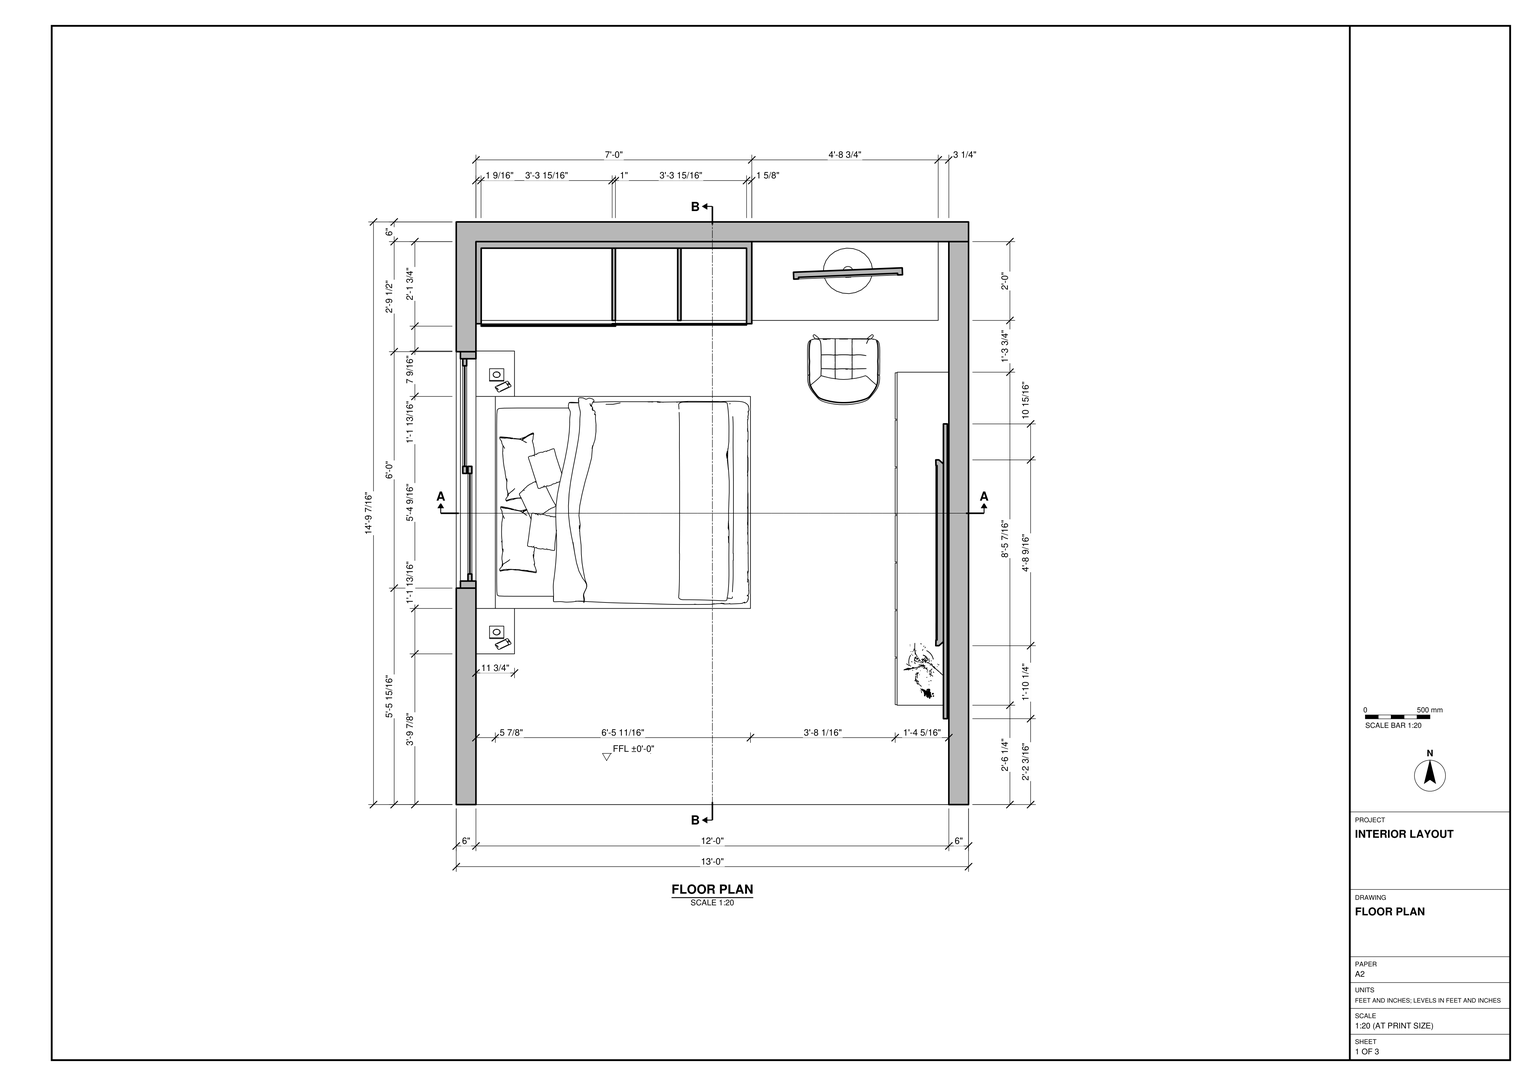
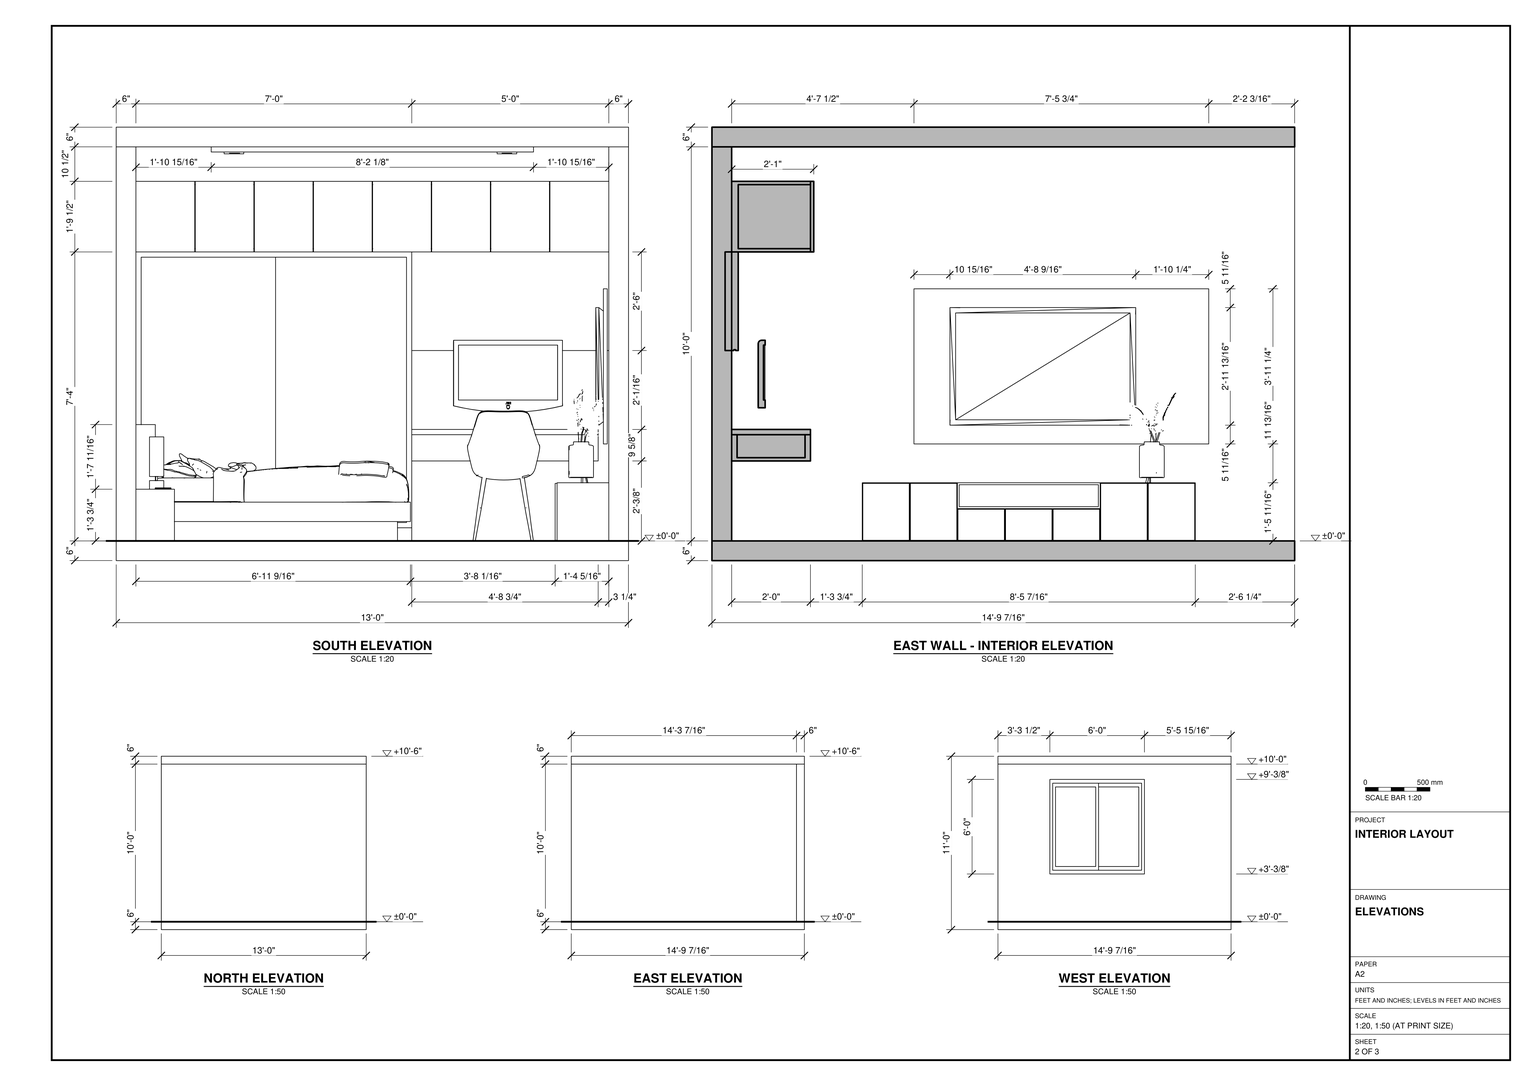
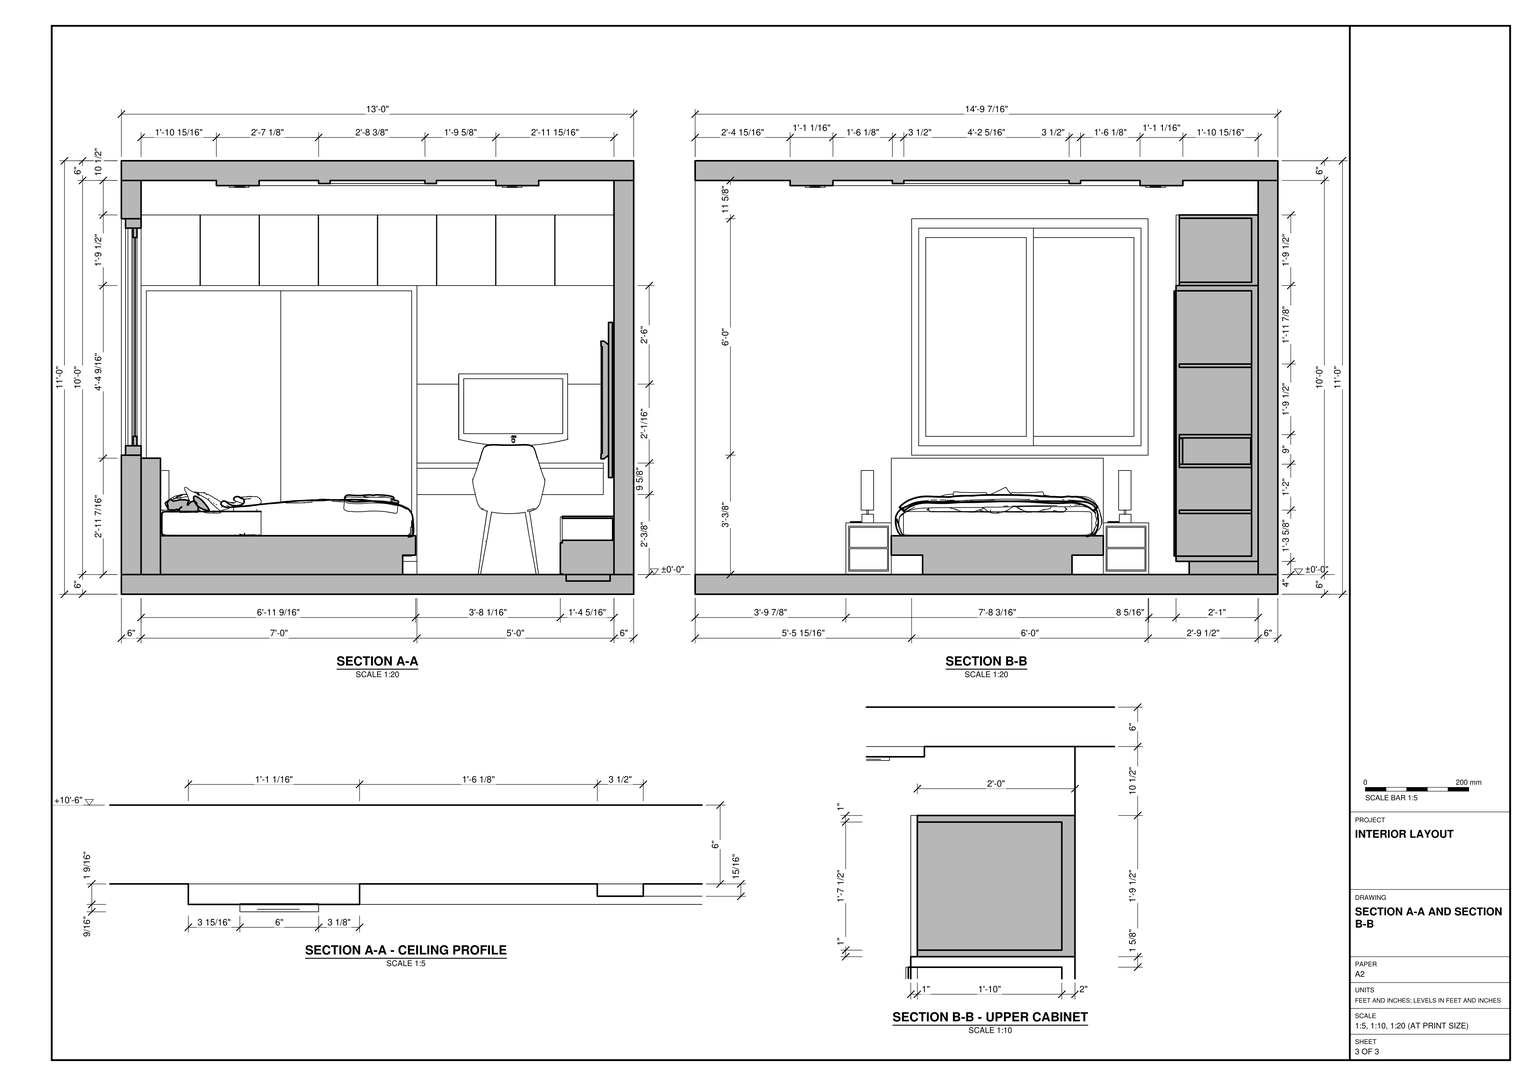
Build the bedroom interior in SketchUp from task_files/diagram_01.pdf. Work in feet and inches. Use the floor plan to set out the room and the elevations and sections to establish heights. The overall dimensions are 13'-0" east to west, 14'-9 7/16" north to south and 11'-0" high. Set the finished floor at ±0'-0". Model the floor slab, the north, east and west walls, and the flat roof slab, leaving the south side open as drawn. Follow the enlarged section for the stepped ceiling profile.

Place the head of the platform bed beneath the framed west window, with a bedside table on either side. Along the north wall, fit the tall wardrobe beside the desk and continue the upper cabinets across both. Include the desk screen and chair. Across the aisle from the foot of the bed, model the east-wall television, its backing panel and the low divided cabinet beneath it. Use the plan for the furniture footprints and the interior elevations for the cabinet divisions. Decor and loose items, including bedside lamps, cushions and the arrangement on the low cabinet, may be any suitable library components.

Keep shell elements and individual furniture and joinery pieces in separate groups or components, and use components for repeated parts. Save one SketchUp model as output_files/bedroom_with_fitted_storage_desk_and_television_wall.skp.

# SketchUp Ruby script. Lengths in inches.
U = 1.inch
M = Sketchup.active_model
def pt(a) = Geom::Point3d.new(a.map { |v| v * U })
def face(e, loops, mat)
  f = e.add_face(loops[0].map { |a| pt(a) })
  loops[1..].each { |l| e.add_face(l.map { |a| pt(a) }).erase! }
  f.material = f.back_material = mat if mat
  f
end
# faces: each face lists its corners as indices into pts; further lists are holes
def faces(e, pts, list, mat = nil) = list.each { |f| face(e, (f[0].is_a?(Array) ? f : [f]).map { |l| l.map { |i| pts[i] } }, mat) }
# xy, xz, yz: faces in a plane at the given z, y or x. An outline is a flat list of corners, or four numbers for a rectangle; further outlines are holes
def ring(l) = l.size == 4 ? [[l[0], l[1]], [l[2], l[1]], [l[2], l[3]], [l[0], l[3]]] : l.each_slice(2).to_a
def flat(e, list, mat, &to3) = list.each { |f| face(e, (f[0].is_a?(Array) ? f : [f]).map { |l| ring(l).map { |u, v| to3.(u, v) } }, mat) }
def xy(e, z, list, mat = nil) = flat(e, list, mat) { |x, y| [x, y, z] }
def xz(e, y, list, mat = nil) = flat(e, list, mat) { |x, z| [x, y, z] }
def yz(e, x, list, mat = nil) = flat(e, list, mat) { |y, z| [x, y, z] }
def lines(e, pts, list) = list.each { |a, b| e.add_line(pt(pts[a]), pt(pts[b])) }
# prism: a flat outline (further loops are holes) pulled along v
def prism(e, loops, v, mat = nil)
  f = face(e, loops, mat); d = Geom::Vector3d.new(v.map { |x| x * U })
  f.pushpull(f.normal.samedirection?(d) ? d.length : -d.length)
end
def box(e, o, s, mat = nil) = prism(e, [[o, [o[0] + s[0], o[1], o[2]], [o[0] + s[0], o[1] + s[1], o[2]], [o[0], o[1] + s[1], o[2]]]], [0, 0, s[2]], mat)
def at(x, y, z, deg = 0) = Geom::Transformation.translation(pt([x, y, z])) * Geom::Transformation.rotation(ORIGIN, Z_AXIS, deg.degrees)
def axes(o, x, y, z) = Geom::Transformation.new([*x, 0, *y, 0, *z, 0, *pt(o).to_a, 1])
def part(name) = M.definitions.add(name)
# library, detail: a bought-in or finely detailed component or shape, given as its bounding box
def library(name, o, s) = part(name).tap { |d| box(d.entities, o, s) }
def detail(e, o, s) = box(e.add_group.entities, o, s)
def put(e, d, t, mat = nil) = e.add_instance(d, t).tap { |i| i.material = mat if mat }
def group(e, t, mat = nil) = e.add_group.tap { |g| g.transformation = t; g.material = mat if mat }.entities
root = M.entities
M.materials.add("[0005_LightPink]").color = [189, 180, 163]
M.materials.add("[0057_DarkKhaki]").color = [189, 183, 107]
M.materials.add("[0092_Azure]").color = [90, 107, 113]
M.materials.add("[Color A01]").color = [96, 100, 74]
M.materials.add("[Color A03]").color = [146, 98, 60]
M.materials.add("[Color A03]1").color = [255, 101, 101]
M.materials.add("[Color H07]").color = [0, 153, 153]
M.materials.add("[Color H08]").color = [0, 102, 102]
M.materials.add("[Color M00]").color = [255, 255, 255]
M.materials.add("[CoolGray4]").color = [225, 226, 230]
M.materials["[CoolGray4]"].alpha = 0.26
M.materials.add("[Field Square Tile]").color = [217, 201, 169]
M.materials.add("[Mirror 02]").color = [229, 229, 229]
M.materials.add("[Roofing Slate Tan]").color = [200, 175, 128]
M.materials.add("[Translucent Glass Blue]").color = [100, 149, 237]
M.materials["[Translucent Glass Blue]"].alpha = 0.5
M.materials.add("[Wood Bamboo]").color = [177, 105, 43]
M.materials.add("[Wood Cherry Original]1").color = [152, 86, 42]
M.materials.add("[Wood Veneer 02]").color = [190, 128, 91]
c1 = part("Cabinet shelf")
box(c1.entities,[0,0,0],[39.93,22,1])
c2 = part("Drawer box")
g1 = group(c2.entities,at(0,1.6875,0))
xy(g1,0,[[0,0,0,22,1,22,1,1,18.96,1,18.96,22,19.96,22,19.96,0],[1,21.75,18.96,22]],"[Wood Veneer 02]")
xy(g1,7.625,[[1,21.75,18.96,22]],"[Wood Veneer 02]")
xy(g1,7.8125,[[0,0,19.96,0,19.96,22,18.96,22,18.96,1,1,1,1,22,0,22]],"[Wood Veneer 02]")
xz(g1,0,[[0,0,19.96,7.8125]],"[Wood Veneer 02]")
xz(g1,1,[[1,0,18.96,7.8125]],"[Wood Veneer 02]")
xz(g1,21.75,[[1,0,18.96,7.625]],"[Wood Veneer 02]")
xz(g1,22,[[0,0,1,7.8125],[1,0,18.96,7.625],[18.96,0,19.96,7.8125]],"[Wood Veneer 02]")
yz(g1,0,[[0,0,22,7.8125]],"[Wood Veneer 02]")
yz(g1,1,[[1,0,21.75,7.8125],[21.75,0,22,7.625],[21.75,7.625,22,7.8125]],"[Wood Veneer 02]")
yz(g1,18.96,[[1,0,21.75,7.8125],[21.75,0,22,7.625],[21.75,7.625,22,7.8125]],"[Wood Veneer 02]")
yz(g1,19.96,[[0,0,22,7.8125]],"[Wood Veneer 02]")
c3 = library("pc",[0,0,0],[196.92,471.66,385.83])
c4 = part("Component")
put(c4.entities,c3,at(-98.46,-353.84,0))
c5 = library("1",[-11,-10.66,0],[22,21.32,33.52])
c6 = library("1.1 TV UNIT",[4.49,5.68,0],[124.23,70.56,78.75])
c7 = library("Double bed",[0,0,0],[83.59,112.46,35.43])
c8 = library("Component\#7",[0,0,0],[6,6,0.625])
c9 = part("Window sash")
g2 = group(c9.entities,at(0.98,0,0))
prism(g2,[[[-0.98,0,0],[30.98,0,0],[30.98,0,45.6],[-0.98,0,45.6]],[[29.01,0,43.625],[29.01,0,1.97],[0.98,0,1.97],[0.98,0,43.625]]],[0,1.18,0])
g3 = group(c9.entities,at(1.97,0.59,1.97),"[Translucent Glass Blue]")
xz(g3,0,[[0,0,28.03,41.66]],"[CoolGray4]")
c10 = part("Two-panel window")
put(c10.entities,c9,at(31.97,2.82,1.97),"[Wood Bamboo]")
put(c10.entities,c9,at(1.97,1.25,1.97),"[Wood Bamboo]")
g4 = group(c10.entities,at(0,0,0),"[Wood Bamboo]")
prism(g4,[[[65.9,4.72,0],[0,4.72,0],[0,4.72,49.53],[65.9,4.72,49.53]],[[1.97,4.72,47.5625],[1.97,4.72,1.97],[63.93,4.72,1.97],[63.93,4.72,47.5625]]],[0,-4.72,0])
c11 = part("Union")
prism(c11.entities,[[[39.93,0,21.5],[19.96,0,21.5],[19.96,0,43.8],[18.96,0,43.8],[18.96,0,21.5],[0,0,21.5],[0,0,20.5],[18.96,0,20.5],[18.96,0,0],[19.96,0,0],[19.96,0,20.5],[39.93,0,20.5]]],[0,22,0])
c12 = part("Group\#17")
box(c12.entities,[-1,0,0],[1,22,19.5])
c13 = part("Drawer box \#1")
xy(c13.entities,0,[[0,0,29.3125,14.5]])
xy(c13.entities,1,[[1,1,28.125,13.5]])
xy(c13.entities,8,[[[0,0,29.3125,14.5],[1,1,28.125,13.5]]])
xz(c13.entities,0,[[0,0,29.3125,8]])
xz(c13.entities,1,[[1,1,28.125,8]])
xz(c13.entities,13.5,[[1,1,28.125,8]])
xz(c13.entities,14.5,[[0,0,29.3125,8]])
yz(c13.entities,0,[[0,0,14.5,8]])
yz(c13.entities,1,[[1,1,13.5,8]])
yz(c13.entities,28.125,[[1,1,13.5,8]])
yz(c13.entities,29.3125,[[0,0,14.5,8]])
c14 = part("Wardrobe door panel")
xy(c14.entities,0,[[0,0,40.93,0.375]],"[0005_LightPink]")
xy(c14.entities,80.8,[[0,0,40.93,0.375]],"[0005_LightPink]")
xz(c14.entities,0,[[0,0,40.93,80.8]],"[Translucent Glass Blue]")
xz(c14.entities,0.375,[[0,0,40.93,80.8]],"[0005_LightPink]")
yz(c14.entities,0,[[0,0,0.375,80.8]],"[0005_LightPink]")
yz(c14.entities,40.93,[[0,0,0.375,80.8]],"[Translucent Glass Blue]")
put(root,c1,at(48.47,147.4375,32.6))
put(root,c2,at(68.4375,145.75,33.6))
put(root,c1,at(7.55,147.4375,32.6))
put(root,c4,axes([110.98,162.19,33.95],[-0.00283,0.07034,0],[-0.07034,-0.00283,0],[0,0,0.0704]))
put(root,c5,axes([117.96,132.4375,0],[1,0,0],[0,-1,0],[0,0,1.18286]))
put(root,c6,at(98.66,136.16,-1.97,-90))
put(root,c7,axes([89.59,45.9,0],[-1,0,0],[0,0.82,0],[0,0,1]))
put(root,c8,at(32.85,33.57,117.875))
put(root,c8,at(32.85,137.19,117.875))
put(root,c8,at(115.98,33.57,117.875))
put(root,c8,at(115.98,137.19,117.875))
g5 = group(root,at(150,21.4375,0),"[0005_LightPink]")
box(g5,[0,-21.4375,0],[6,171.4375,120])
g6 = group(root,at(0,21.4375,-6),"[Roofing Slate Tan]")
box(g6,[0,-21.4375,0],[156,177.4375,6],"[Field Square Tile]")
g7 = group(root,at(0,21.4375,0),"[0057_DarkKhaki]")
xy(g7,0,[[0,-21.4375,0,156,156,156,156,150,6,150,6,-21.4375]],"[Color A01]")
xy(g7,36.35,[[0,44.49,6,116.49]],"[Color A01]")
xy(g7,108.35,[[0,44.49,6,116.49]],"[Color A01]")
xy(g7,120,[[0,-21.4375,6,-21.4375,6,150,156,150,156,156,0,156]],"[0005_LightPink]")
xz(g7,-21.4375,[[0,0,6,120]],"[0005_LightPink]")
xz(g7,44.49,[[0,36.35,6,108.35]],"[Color A01]")
xz(g7,116.49,[[0,36.35,6,108.35]],"[Color A01]")
xz(g7,150,[[6,0,156,120]],"[0005_LightPink]")
xz(g7,156,[[0,0,156,120]],"[0005_LightPink]")
yz(g7,0,[[[-21.4375,0,156,120],[44.49,36.35,116.49,108.35]]],"[0005_LightPink]")
yz(g7,6,[[[-21.4375,0,150,120],[44.49,36.35,116.49,108.35]]],"[Color A01]")
yz(g7,156,[[150,0,156,120]],"[0005_LightPink]")
put(g7,c10,axes([6,44.49,36.35],[0,1.09255,0],[-1,0,0],[0,0,1.45359]),"[Wood Cherry Original]1")
g8 = group(root,at(6,145.75,0),"[Color M00]")
put(g8,c2,at(42.47,0,33.6))
put(g8,c2,at(1.55,0,33.6))
put(g8,c2,at(21.51,0,33.6))
put(g8,c1,at(1.55,1.6875,41.6))
put(g8,c1,at(42.47,1.6875,41.6))
put(g8,c1,at(1.55,1.6875,18.6))
put(g8,c1,at(42.47,1.6875,18.6))
g9 = group(g8,at(0,1.6875,0),"[0005_LightPink]")
g10 = group(g9,at(0,0,0))
box(g10,[0,3,0],[84,21,4])
g11 = group(g9,at(0,0,4))
xy(g11,0,[[0,-1,84,24]])
xy(g11,1.6,[[1.6,-1,42.47,22],[42.47,-1,82.4,22]])
xy(g11,82.4,[[1.6,-1,82.4,22]])
xy(g11,84,[[0,-1,84,24]])
xz(g11,-1,[[[0,0,84,84],[1.6,1.6,82.4,82.4]]])
xz(g11,22,[[1.6,1.6,82.4,82.4]])
xz(g11,24,[[0,0,84,84]])
yz(g11,0,[[-1,0,24,84]])
yz(g11,1.6,[[-1,1.6,22,82.4]])
yz(g11,82.4,[[-1,1.6,22,82.4]])
yz(g11,84,[[-1,0,24,84]])
g12 = group(g8,at(41.47,1.6875,5.6))
prism(g12,[[[1,0,37],[1,0,80.8],[0,0,80.8],[0,0,0],[1,0,0]]],[0,22,0])
put(g8,c11,at(42.47,1.6875,42.6))
g13 = group(root,at(6,147.4375,88),"[Wood Veneer 02]")
xy(g13,0,[[0,0,144,24]],"[0005_LightPink]")
xy(g13,1,[[1,0,143,22]])
xy(g13,20.5,[[1,0,143,22]])
xy(g13,21.5,[[0,0,144,24]],"[0005_LightPink]")
xz(g13,0,[[[0,0,144,21.5],[1,1,143,20.5]]])
xz(g13,22,[[1,1,143,20.5]],"[Color H08]")
xz(g13,24,[[0,0,144,21.5]])
yz(g13,0,[[0,0,24,21.5]])
yz(g13,1,[[0,1,22,20.5]])
yz(g13,143,[[0,1,22,20.5]])
yz(g13,144,[[0,0,24,21.5]],"[0005_LightPink]")
put(root,c12,at(42.75,147.4375,89))
put(root,c12,at(78.5,147.4375,89))
put(root,c12,at(114.25,147.4375,89))
g14 = group(root,at(6,146.4375,88),"[Color A01]")
box(g14,[90.08,0,0],[17.84,1,21.5],"[0005_LightPink]")
xy(g14,0,[[0,0,17.92,1],[18.08,0,35.92,1],[36.08,0,53.92,1],[54.08,0,71.92,1],[72.08,0,89.92,1],
  [108.08,0,125.92,1]])
xy(g14,0,[[126.08,0,144,1]],"[Color H08]")
xy(g14,21.5,[[0,0,17.92,1],[18.08,0,35.92,1],[36.08,0,53.92,1],[54.08,0,71.92,1],[72.08,0,89.92,1],
  [108.08,0,125.92,1]])
xy(g14,21.5,[[126.08,0,144,1]],"[Color H08]")
xz(g14,0,[[0,0,17.92,21.5],[18.08,0,35.92,21.5],[36.08,0,53.92,21.5],[54.08,0,71.92,21.5],[72.08,0,89.92,21.5],
  [108.08,0,125.92,21.5],[126.08,0,144,21.5]],"[0005_LightPink]")
xz(g14,1,[[0,0,17.92,21.5],[18.08,0,35.92,21.5],[36.08,0,53.92,21.5],[54.08,0,71.92,21.5],[72.08,0,89.92,21.5],
  [108.08,0,125.92,21.5]])
xz(g14,1,[[126.08,0,144,21.5]],"[Color H08]")
yz(g14,0,[[0,0,1,21.5]])
yz(g14,17.92,[[0,0,1,21.5]])
yz(g14,18.08,[[0,0,1,21.5]])
yz(g14,35.92,[[0,0,1,21.5]])
yz(g14,36.08,[[0,0,1,21.5]])
yz(g14,53.92,[[0,0,1,21.5]])
yz(g14,54.08,[[0,0,1,21.5]])
yz(g14,71.92,[[0,0,1,21.5]])
yz(g14,72.08,[[0,0,1,21.5]])
yz(g14,89.92,[[0,0,1,21.5]])
yz(g14,108.08,[[0,0,1,21.5]])
yz(g14,125.92,[[0,0,1,21.5]])
yz(g14,126.08,[[0,0,1,21.5]],"[Color H08]")
yz(g14,144,[[0,0,1,21.5]],"[Color H08]")
g15 = group(root,at(90,156.9375,24.35))
put(g15,c13,axes([0,-9.5,0],[0.9651,0,0],[0,1.65517,0],[0,0,1]),"[Wood Veneer 02]")
put(g15,c13,axes([28.47,-9.5,0],[0.9651,0,0],[0,1.65517,0],[0,0,1]),"[Wood Veneer 02]")
g16 = group(g15,at(0,-9.5,8),"[0005_LightPink]")
prism(g16,[[[0,0,0],[28.95,0,0],[56.76,0,0],[56.76,0,1.6],[0,0,1.6]]],[0,24,0])
g17 = group(root,at(90,171.4375,57.98),"[Color A03]")
xy(g17,0,[[0,-2,60,-1.22],[0,-0.64,60,2]])
xy(g17,0.25,[[0,-1.22,60,-0.64]])
xy(g17,30.02,[[0,-2,60,2]])
xz(g17,-2,[[0,0,60,30.02]],"[0092_Azure]")
xz(g17,-1.22,[[0,0,60,0.25]])
xz(g17,-0.64,[[0,0,60,0.25]])
xz(g17,2,[[0,0,60,30.02]])
yz(g17,0,[[-2,0,-2,30.02,2,30.02,2,0,-0.64,0,-0.64,0.25,-1.22,0.25,-1.22,0]])
yz(g17,60,[[-2,0,-1.22,0,-1.22,0.25,-0.64,0.25,-0.64,0,2,0,2,30.02,-2,30.02]])
g18 = group(root,at(48.47,145.6875,5.6),"[Mirror 02]")
put(g18,c14,at(-1,0.375,0),"[0005_LightPink]")
put(g18,c14,at(-40.875,0,0))
g19 = group(root,at(0,0,120))
xy(g19,-1.5625,[[[28.93,28.93,127.07,148.51],[41.96,41.96,114.04,135.47]]],"[Color A03]1")
xy(g19,-0.9375,[[[60.06,60.06,95.94,117.38],[63.56,63.56,92.44,113.88]]],"[Color H07]")
xy(g19,0,[[[0,0,156,177.4375],[28.93,28.93,127.07,148.51]],[[41.96,41.96,114.04,135.47],[60.06,60.06,95.94,117.38]],[63.56,63.56,92.44,113.88]],"[0005_LightPink]")
xy(g19,6,[[0,0,156,177.4375]],"[0005_LightPink]")
xz(g19,0,[[0,0,156,6]],"[0005_LightPink]")
xz(g19,28.93,[[28.93,-1.5625,127.07,0]],"[Color A03]1")
xz(g19,41.96,[[41.96,-1.5625,114.04,0]],"[0005_LightPink]")
xz(g19,60.06,[[60.06,-0.9375,95.94,0]],"[Color H07]")
xz(g19,63.56,[[63.56,-0.9375,92.44,0]],"[0005_LightPink]")
xz(g19,113.88,[[63.56,-0.9375,92.44,0]],"[Color H07]")
xz(g19,117.38,[[60.06,-0.9375,95.94,0]],"[0005_LightPink]")
xz(g19,135.47,[[41.96,-1.5625,114.04,0]],"[Color A03]1")
xz(g19,148.51,[[28.93,-1.5625,127.07,0]],"[0005_LightPink]")
xz(g19,177.4375,[[0,0,156,6]],"[0005_LightPink]")
yz(g19,0,[[0,0,177.4375,6]],"[0005_LightPink]")
yz(g19,28.93,[[28.93,-1.5625,148.51,0]],"[Color A03]1")
yz(g19,41.96,[[41.96,-1.5625,135.47,0]],"[Color A03]1")
yz(g19,60.06,[[60.06,-0.9375,117.38,0]],"[Color H07]")
yz(g19,63.56,[[63.56,-0.9375,113.88,0]],"[Color H07]")
yz(g19,92.44,[[63.56,-0.9375,113.88,0]],"[Color H07]")
yz(g19,95.94,[[60.06,-0.9375,117.38,0]],"[Color H07]")
yz(g19,114.04,[[41.96,-1.5625,135.47,0]],"[Color A03]1")
yz(g19,127.07,[[28.93,-1.5625,148.51,0]],"[Color A03]1")
yz(g19,156,[[0,0,177.4375,6]],"[0005_LightPink]")
